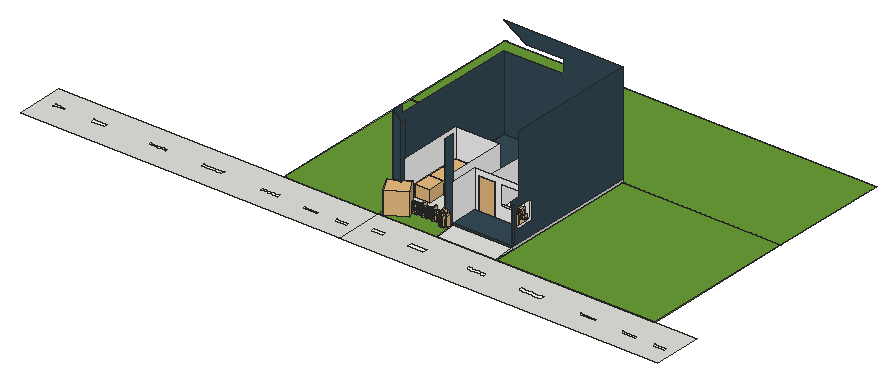
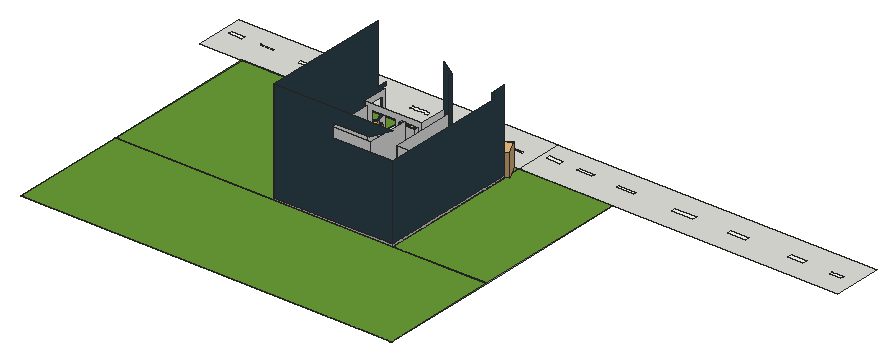
# SketchUp Ruby script. Lengths in inches.
U = 1.inch
M = Sketchup.active_model
def pt(a) = Geom::Point3d.new(a.map { |v| v * U })
def face(e, loops, mat)
  f = e.add_face(loops[0].map { |a| pt(a) })
  loops[1..].each { |l| e.add_face(l.map { |a| pt(a) }).erase! }
  f.material = f.back_material = mat if mat
  f
end
# faces: each face lists its corners as indices into pts; further lists are holes
def faces(e, pts, list, mat = nil) = list.each { |f| face(e, (f[0].is_a?(Array) ? f : [f]).map { |l| l.map { |i| pts[i] } }, mat) }
# xy, xz, yz: faces in a plane at the given z, y or x. An outline is a flat list of corners, or four numbers for a rectangle; further outlines are holes
def ring(l) = l.size == 4 ? [[l[0], l[1]], [l[2], l[1]], [l[2], l[3]], [l[0], l[3]]] : l.each_slice(2).to_a
def flat(e, list, mat, &to3) = list.each { |f| face(e, (f[0].is_a?(Array) ? f : [f]).map { |l| ring(l).map { |u, v| to3.(u, v) } }, mat) }
def xy(e, z, list, mat = nil) = flat(e, list, mat) { |x, y| [x, y, z] }
def xz(e, y, list, mat = nil) = flat(e, list, mat) { |x, z| [x, y, z] }
def yz(e, x, list, mat = nil) = flat(e, list, mat) { |y, z| [x, y, z] }
def lines(e, pts, list) = list.each { |a, b| e.add_line(pt(pts[a]), pt(pts[b])) }
# prism: a flat outline (further loops are holes) pulled along v
def prism(e, loops, v, mat = nil)
  f = face(e, loops, mat); d = Geom::Vector3d.new(v.map { |x| x * U })
  f.pushpull(f.normal.samedirection?(d) ? d.length : -d.length)
end
def box(e, o, s, mat = nil) = prism(e, [[o, [o[0] + s[0], o[1], o[2]], [o[0] + s[0], o[1] + s[1], o[2]], [o[0], o[1] + s[1], o[2]]]], [0, 0, s[2]], mat)
def at(x, y, z, deg = 0) = Geom::Transformation.translation(pt([x, y, z])) * Geom::Transformation.rotation(ORIGIN, Z_AXIS, deg.degrees)
def axes(o, x, y, z) = Geom::Transformation.new([*x, 0, *y, 0, *z, 0, *pt(o).to_a, 1])
def part(name) = M.definitions.add(name)
# library, detail: a bought-in or finely detailed component or shape, given as its bounding box
def library(name, o, s) = part(name).tap { |d| box(d.entities, o, s) }
def detail(e, o, s) = box(e.add_group.entities, o, s)
def put(e, d, t, mat = nil) = e.add_instance(d, t).tap { |i| i.material = mat if mat }
def group(e, t, mat = nil) = e.add_group.tap { |g| g.transformation = t; g.material = mat if mat }.entities
root = M.entities
M.materials.add("0496 AP 9691 Shadow-N").color = [53, 75, 86]
M.materials.add("Color_1").color = [255, 255, 255]
M.materials.add("POT_TEXTURE_1").color = [172, 172, 172]
M.materials.add("[Color M00]").color = [255, 255, 255]
M.materials.add("[Grass Dark Green]").color = [106, 157, 55]
M.materials.add("skp avat flo 1").color = [0, 129, 229]
M.materials.add("skp avat flo 2").color = [47, 120, 22]
M.materials.add("soil1").color = [68, 55, 47]
c1 = library("ruselia",[-5.83,-15.14,-32.53],[55.24,20.14,57.16])
c2 = part("Untitled")
xy(c2.entities,0,[[[158.81,26.5625,306.06,993.3125],[226.57,518.17,239.57,583.92],[225.28,357.51,237.28,411.51],[222.61,182.28,236.36,226.53],[239.71,931.55,251.46,972.3],[233.64,703.93,242.14,755.18],[240.05,835.03,248.8,880.53],[222.04,66.5,231.29,100.5]]])
xy(c2.entities,0,[[222.04,66.5,231.29,100.5],[222.61,182.28,236.36,226.53],[225.28,357.51,237.28,411.51],[226.57,518.17,239.57,583.92],[233.64,703.93,242.14,755.18],
  [240.05,835.03,248.8,880.53],[239.71,931.55,251.46,972.3]],"Color_1")
c3 = library("Cay chuoi",[-26.05,-21.66,0],[63.57,52.43,69.02])
c4 = library("Group\#146",[-640.625,-1318.37,287.11],[396.64,314.81,689.96])
c5 = library("Group\#133",[-513.94,-1201.2,195.17],[480.66,557.42,1160.08])
c6 = library("Group\#135",[-208.03,-1336.63,286.21],[381.72,484.79,1145.39])
c7 = library("Group\#149",[-619.83,-1636.3,288.9],[316.15,456.61,1171.28])
c8 = library("Group\#150",[-738.91,-1210.08,301],[426.4,388.88,1000.79])
c9 = library("Group\#152",[-208.33,-1511.76,297.04],[508.2,421.96,1258.76])
c10 = library("Group\#134",[-545.36,-1775.03,287.125],[412.21,432,920.68])
c11 = library("Group\#147",[-750.24,-1478.51,301.56],[423.84,451.05,998.69])
c12 = library("Group\#137",[-245.33,-1174.2,301.22],[356.02,306.31,608.34])
c13 = library("Group\#132",[-487.23,-1483.58,-4.71],[450.86,446.99,418.38])
c14 = library("Group\#154",[-445.7,-1606.55,154.18],[255.44,283.57,849.28])
c15 = library("Group\#155",[-390.1,-1177.12,195.59],[220.93,265.44,790.12])
c16 = library("Group\#157",[-480.32,-1333.42,295.8],[424.49,356.06,1482.77])
c17 = library("Group\#158",[-378.01,-1245.98,305.66],[422.15,474.55,1267.42])
c18 = library("Group\#136",[-163.65,-1622.09,292.29],[406.18,374.8,780.12])
c19 = library("Group\#153",[-384.8,-1640.99,300.61],[422.68,348.03,1297.96])
c20 = library("Group\#131",[-373.85,-1441.17,362.05],[290.51,348.28,45.35])
c21 = library("Group\#156",[-208.0625,-1498.77,286.27],[547.26,435.76,1075.6])
c22 = library("Group\#151",[-172.82,-1329.68,294.68],[502.85,397.72,955.79])
c23 = library("Group\#148",[-426.76,-1753.59,287.48],[479.67,412.35,1049.19])
c24 = part("Potted palm")
put(c24.entities,c4,axes([750.24,1775.03,-132.93],[1,0,0],[0,1,0],[0,0,1.2036]))
put(c24.entities,c5,axes([750.24,1775.03,-132.93],[1,0,0],[0,1,0],[0,0,1.2036]))
put(c24.entities,c6,axes([750.24,1775.03,-132.93],[1,0,0],[0,1,0],[0,0,1.2036]))
put(c24.entities,c7,axes([750.24,1775.03,-132.93],[1,0,0],[0,1,0],[0,0,1.2036]))
put(c24.entities,c8,axes([750.24,1775.03,-132.93],[1,0,0],[0,1,0],[0,0,1.2036]))
put(c24.entities,c9,axes([750.24,1775.03,-132.93],[1,0,0],[0,1,0],[0,0,1.2036]))
put(c24.entities,c10,axes([750.24,1775.03,-132.93],[1,0,0],[0,1,0],[0,0,1.2036]))
put(c24.entities,c11,axes([750.24,1775.03,-132.93],[1,0,0],[0,1,0],[0,0,1.2036]))
put(c24.entities,c12,axes([750.24,1775.03,-132.93],[1,0,0],[0,1,0],[0,0,1.2036]))
put(c24.entities,c13,axes([746.24,1775.03,3.02],[0.89,0,0],[0,1,0],[0,0,0.64]),"POT_TEXTURE_1")
put(c24.entities,c14,axes([750.24,1775.03,-132.93],[1,0,0],[0,1,0],[0,0,1.2036]))
put(c24.entities,c15,axes([750.24,1775.03,-132.93],[1,0,0],[0,1,0],[0,0,1.2036]))
put(c24.entities,c16,axes([750.24,1775.03,-132.93],[1,0,0],[0,1,0],[0,0,1.2036]))
put(c24.entities,c17,axes([750.24,1775.03,-132.93],[1,0,0],[0,1,0],[0,0,1.2036]))
put(c24.entities,c18,axes([750.24,1775.03,-132.93],[1,0,0],[0,1,0],[0,0,1.2036]))
put(c24.entities,c19,axes([750.24,1775.03,-132.93],[1,0,0],[0,1,0],[0,0,1.2036]))
put(c24.entities,c20,at(750.24,1775.03,-101.54),"soil1")
put(c24.entities,c21,axes([750.24,1775.03,-132.93],[1,0,0],[0,1,0],[0,0,1.2036]))
put(c24.entities,c22,axes([750.24,1775.03,-132.93],[1,0,0],[0,1,0],[0,0,1.2036]))
put(c24.entities,c23,axes([750.24,1775.03,-132.93],[1,0,0],[0,1,0],[0,0,1.2036]))
c25 = library("skpD0I6a8",[14.43,-68.68,0],[105.42,143.14,64.75])
c26 = library("skp0QfVtK",[14.45,-36.06,-0.05],[111.77,111,64.8])
c27 = library("skpcyxm1p",[14.43,-75.28,0],[105.19,111.11,34.48])
c28 = library("Sectional sofa module",[0,0,0],[105.41,111.76,64.75])
c29 = part("L Shaped Sofa (30)")
put(c29.entities,c25,at(757.73,0.41,0))
put(c29.entities,c26,axes([685.96,0.19,0],[-1,0,0],[0,1,0],[0,0,1]))
put(c29.entities,c27,at(605.64,-125.1875,0))
put(c29.entities,c28,axes([669.02,-36.11,0],[1,0,0],[0,0.99,0],[0,0,1]))
c30 = library("Group\#97",[-662.41,217.3,320.04],[397.32,658.3,1732.06])
c31 = library("Group\#99",[-299.2,181.55,262.58],[360.65,735.71,1258.34])
c32 = library("Group\#94",[-1038.76,656.55,345.34],[733.18,460.51,2065.7])
c33 = library("Group\#92",[-445.29,890.31,329.28],[284.3,304.08,2023.29])
c34 = library("Group\#95",[-733.48,439.625,202.64],[456.28,533.12,1536.78])
c35 = library("Group\#98",[-455.56,899.32,410.78],[341.21,610.33,1581.5])
c36 = library("Group\#91",[-516.34,626.77,-4.5625],[517.73,515.95,418.98])
c37 = library("Group\#96",[-249.24,914.85,310.18],[345.55,647.95,1307.93])
c38 = library("Group\#93",[-277.97,488.68,287.26],[362.84,405.94,1768.54])
c39 = library("Group\#90",[-468.76,669.89,380.1875],[424.36,427.47,41.99])
c40 = part("Potted tropical plant")
put(c40.entities,c30,at(1038.76,-181.55,4.5625))
put(c40.entities,c31,at(1038.76,-181.55,4.5625))
put(c40.entities,c32,at(1038.76,-181.55,4.5625))
put(c40.entities,c33,at(1038.76,-181.55,4.5625))
put(c40.entities,c34,at(1038.76,-181.55,4.5625))
put(c40.entities,c35,at(1038.76,-181.55,4.5625))
put(c40.entities,c36,at(1038.76,-181.55,4.5625),"POT_TEXTURE_1")
put(c40.entities,c37,at(1038.76,-181.55,4.5625))
put(c40.entities,c38,at(1038.76,-181.55,4.5625))
put(c40.entities,c39,at(1038.76,-181.55,4.5625),"soil1")
c41 = library("door by lz",[5.91,-4.92,0],[35.43,6.61,78.74])
c42 = part("Gruppe\#2")
xy(c42.entities,0,[[6.69,0,4.96,0.23,3.03,1.59,1.96,1.96,0.9,3.35,0.9,5.71,0,6.69,0.23,8.43,1.96,10,3.35,12.49,4.67,13.04,7.04,12.49,8.72,13.04,10.04,12.49,11.43,11.43,12.05,9.15,13.39,6.69,13.16,4.96,12.49,3.35,10.41,2.22,8.43,0.23]],"skp avat flo 1")
c43 = part("Gruppe\#12")
xy(c43.entities,0,[[1.18,0.5,1.36,0.52,1.52,0.59,1.67,0.7,1.77,0.84,1.84,1,1.87,1.18,1.84,1.36,1.77,1.52,1.67,1.67,1.52,1.77,1.36,1.84,1.18,1.87,1,1.84,0.84,1.77,0.7,1.67,0.59,1.52,0.52,1.36,0.5,1.18,0.52,1,0.59,0.84,0.7,0.7,0.84,0.59,1,0.52]])
c44 = part("f.st. wop plant 01 blüte")
put(c44.entities,c42,at(0,0,0))
put(c44.entities,c43,at(5.65,5.41,0.39))
c45 = part("Gruppe\#5")
xy(c45.entities,0.96,[[13.97,0.22,8.73,4.42,7.37,10.11,8.43,14.53,13.97,16.39]],"skp avat flo 2")
p = [[13.97,0.22,0.96],[13.97,16.39,0.96],[17.89,14.53,4.875],[18.64,10.11,5.625],[17.67,4.42,4.66]]
faces(c45.entities,p,[[0,1,2,3,4]],"skp avat flo 2")
c46 = part("f.st. wop plant 01 blatt")
put(c46.entities,c45,axes([0.99,0,4.74],[0.91566,0,-0.40195],[0,1,0],[0.40195,0,0.91566]))
c47 = part("Gruppe\#10")
put(c47.entities,c44,axes([4.61,0.45,57.14],[0.99373,-0.06775,-0.08889],[0.11172,0.62588,0.77188],[0.00335,-0.77697,0.62953]))
put(c47.entities,c44,axes([12.4,0.4,0.59],[0.70061,0.70799,-0.08889],[-0.40079,0.49353,0.77188],[0.59035,-0.50516,0.62953]))
put(c47.entities,c44,axes([24.4375,6.09,17.58],[-0.05734,0.99439,-0.08889],[-0.63495,0.03239,0.77188],[0.77043,0.1007,0.62953]))
put(c47.entities,c44,axes([1.11,8.09,13.25],[0.88983,-0.44754,-0.08889],[0.34553,0.53368,0.77188],[-0.298,-0.71756,0.62953]))
put(c47.entities,c44,axes([23.26,15,37.53],[-0.84836,0.52191,-0.08889],[-0.38985,-0.50222,0.77188],[0.35821,0.68948,0.62953]))
put(c47.entities,c44,axes([12.67,23.61,24.88],[-0.75852,-0.64555,-0.08889],[0.35717,-0.52596,0.77188],[-0.54504,0.55374,0.62953]))
put(c47.entities,c44,axes([20.43,22.9,81.42],[-0.98432,0.15238,-0.08889],[-0.16477,-0.61405,0.77188],[0.06303,0.77442,0.62953]))
put(c47.entities,c44,axes([1.76,2.9,29.21],[0.93833,-0.33412,-0.08889],[0.27691,0.5723,0.77188],[-0.20703,-0.74889,0.62953]))
put(c47.entities,c44,axes([13.59,0.5,77.09],[0.62412,0.77625,-0.08889],[-0.4494,0.44972,0.77188],[0.63915,-0.4418,0.62953]))
put(c47.entities,c44,axes([-1.26,15.51,69.79],[0.24265,-0.96603,-0.08889],[0.62977,0.08716,0.77188],[-0.73791,-0.24328,0.62953]))
put(c47.entities,c44,axes([22.04,17.92,65.46],[-0.95793,0.27287,-0.08889],[-0.2394,-0.58898,0.77188],[0.15827,0.76069,0.62953]))
put(c47.entities,c44,axes([9.51,23.35,52.81],[-0.55554,-0.82673,-0.08889],[0.48617,-0.40969,0.77188],[-0.67455,0.38559,0.62953]))
put(c47.entities,c44,axes([0.1875,18.97,41.86],[-0.02781,-0.99565,-0.08889],[0.62986,-0.08651,0.77188],[-0.77621,-0.03452,0.62953]))
put(c47.entities,c44,axes([24.98,7.4,94.08],[-0.15925,0.98323,-0.08889],[-0.63491,-0.03305,0.77188],[0.75599,0.17936,0.62953]))
put(c47.entities,c44,axes([21.5,21.98,4.93],[-0.96344,0.25275,-0.08889],[-0.22702,-0.59386,0.77188],[0.1423,0.76384,0.62953]))
put(c47.entities,c44,axes([1.57,6.98,89.75],[0.93112,-0.3537,-0.08889],[0.28884,0.56637,0.77188],[-0.22267,-0.74439,0.62953]))
put(c47.entities,c46,axes([9.37,32.32,90.95],[-0.51317,-0.65235,0],[0.5996,-0.47167,0.32697],[-0.25699,0.20216,0.76288]))
put(c47.entities,c46,axes([33.81,6.72,78.35],[-0.27992,0.78137,0],[-0.71819,-0.25729,0.32697],[0.30782,0.11027,0.76288]))
put(c47.entities,c46,axes([-9.46,14.86,61.47],[0.53029,-0.63851,0],[0.58688,0.4874,0.32697],[-0.25154,-0.2089,0.76288]))
put(c47.entities,c46,axes([21.49,-6.15,66.98],[0.2591,0.78852,0],[-0.72476,0.23815,0.32697],[0.31063,-0.10207,0.76288]))
put(c47.entities,c46,axes([32.03,5.27,54.38],[-0.36397,0.74594,0],[-0.68562,-0.33454,0.32697],[0.29386,0.14338,0.76288]))
put(c47.entities,c46,axes([30.63,20.6,49.31],[-0.77544,0.29596,0],[-0.27203,-0.71273,0.32697],[0.11659,0.30548,0.76288]))
put(c47.entities,c46,axes([32.03,5.27,27.16],[-0.36397,0.74594,0],[-0.68562,-0.33454,0.32697],[0.29386,0.14338,0.76288]))
put(c47.entities,c46,axes([17.4375,27.53,13.8125],[-0.76735,-0.23527,0.21148],[0.29408,-0.735,0.24937],[0.11659,0.30548,0.76288]))
put(c47.entities,c46,axes([-9.46,14.86,34.24],[0.53029,-0.63851,0],[0.58688,0.4874,0.32697],[-0.25154,-0.2089,0.76288]))
c48 = part("Gruppe\#9")
put(c48.entities,c44,axes([2.2,1.62,57.61],[0.97169,-0.0623,-0.22792],[0.22172,0.57378,0.78843],[0.08166,-0.81664,0.57134]))
put(c48.entities,c44,axes([-1.48,7.53,1.27],[0.68093,0.71536,-0.15682],[-0.22028,0.40428,0.88771],[0.69843,-0.56993,0.43287]))
put(c48.entities,c44,axes([13.97,11.34,15.86],[-0.0542,0.99797,0.03349],[-0.45869,-0.05467,0.88691],[0.88694,0.03271,0.46072]))
put(c48.entities,c44,axes([-9.71,13.74,16.77],[0.84218,-0.4326,-0.32186],[0.5102,0.4462,0.73526],[-0.17446,-0.78343,0.59649]))
put(c48.entities,c44,axes([17.17,17.99,36.46],[-0.83727,0.52624,0.14846],[-0.23006,-0.58536,0.77745],[0.49603,0.61679,0.61117]))
put(c48.entities,c44,axes([4.35,27.92,27.32],[-0.77345,-0.63385,0.00301],[0.4998,-0.60694,0.61792],[-0.38984,0.47943,0.78623]))
put(c48.entities,c44,axes([20.43,22.9,81.42],[-0.98432,0.15238,-0.08889],[-0.16477,-0.61405,0.77188],[0.06303,0.77442,0.62953]))
put(c48.entities,c44,axes([-5.84,6.82,31.58],[0.89192,-0.31974,-0.31975],[0.44391,0.4844,0.75386],[-0.08616,-0.81432,0.57398]))
put(c48.entities,c44,axes([13.59,0.5,77.09],[0.62412,0.77625,-0.08889],[-0.4494,0.44972,0.77188],[0.63915,-0.4418,0.62953]))
put(c48.entities,c44,axes([-1.26,15.51,69.79],[0.24265,-0.96603,-0.08889],[0.62977,0.08716,0.77188],[-0.73791,-0.24328,0.62953]))
put(c48.entities,c44,axes([20.77,18.5,64.59],[-0.95848,0.27864,0.06062],[-0.13765,-0.63827,0.75741],[0.24973,0.71762,0.65012]))
put(c48.entities,c44,axes([6.6875,24.75,54.15],[-0.57029,-0.8188,-0.06577],[0.58283,-0.45976,0.67002],[-0.57885,0.34377,0.73942]))
put(c48.entities,c44,axes([-4.08,21.11,44.3125],[-0.04911,-0.98765,-0.14878],[0.72825,-0.13735,0.67141],[-0.68355,-0.07538,0.726]))
put(c48.entities,c44,axes([24.98,7.4,94.08],[-0.15925,0.98323,-0.08889],[-0.63491,-0.03305,0.77188],[0.75599,0.17936,0.62953]))
put(c48.entities,c44,axes([8.77,28.52,5.9],[-0.95532,0.25842,0.14346],[-0.07274,-0.676,0.7333],[0.28648,0.6901,0.6646]))
put(c48.entities,c44,axes([1.57,6.98,89.75],[0.93112,-0.3537,-0.08889],[0.28884,0.56637,0.77188],[-0.22267,-0.74439,0.62953]))
put(c48.entities,c46,axes([9.37,32.32,90.95],[-0.51317,-0.65235,0],[0.5996,-0.47167,0.32697],[-0.25699,0.20216,0.76288]))
put(c48.entities,c46,axes([33.81,6.72,78.35],[-0.27992,0.78137,0],[-0.71819,-0.25729,0.32697],[0.30782,0.11027,0.76288]))
put(c48.entities,c46,axes([-11.01,15.72,64.74],[0.51926,-0.63742,-0.11388],[0.63054,0.46456,0.27478],[-0.14729,-0.25842,0.77487]))
put(c48.entities,c46,axes([20.21,-5.625,64.6],[0.26417,0.78668,0.01588],[-0.67119,0.21655,0.43762],[0.41063,-0.15212,0.70508]))
put(c48.entities,c46,axes([29.04,6.59,51.45],[-0.35348,0.74452,0.09816],[-0.63785,-0.35493,0.39506],[0.39635,0.09281,0.72332]))
put(c48.entities,c46,axes([27.11,22.23,47.625],[-0.76537,0.29574,0.12508],[-0.23173,-0.73252,0.31403],[0.22228,0.25465,0.75805]))
put(c48.entities,c46,axes([23.375,9.49,23.48],[-0.34051,0.7404,0.15735],[-0.60881,-0.37042,0.42548],[0.44978,0.05914,0.69506]))
put(c48.entities,c46,axes([6.77,33.04,15.99],[-0.71083,-0.25923,0.3412],[0.32455,-0.75723,0.10082],[0.2798,0.21977,0.74988]))
put(c48.entities,c46,axes([-15.51,18.125,40.12],[0.50532,-0.63318,-0.18065],[0.65217,0.44994,0.24724],[-0.09068,-0.29247,0.77145]))
c49 = part("Gruppe\#11")
put(c49.entities,c44,axes([4.61,0.45,57.14],[0.99373,-0.06775,-0.08889],[0.11172,0.62588,0.77188],[0.00335,-0.77697,0.62953]))
put(c49.entities,c44,axes([12.4,0.4,0.59],[0.70061,0.70799,-0.08889],[-0.40079,0.49353,0.77188],[0.59035,-0.50516,0.62953]))
put(c49.entities,c44,axes([24.4375,6.09,17.58],[-0.05734,0.99439,-0.08889],[-0.63495,0.03239,0.77188],[0.77043,0.1007,0.62953]))
put(c49.entities,c44,axes([1.11,8.09,13.25],[0.88983,-0.44754,-0.08889],[0.34553,0.53368,0.77188],[-0.298,-0.71756,0.62953]))
put(c49.entities,c44,axes([23.26,15,37.53],[-0.84836,0.52191,-0.08889],[-0.38985,-0.50222,0.77188],[0.35821,0.68948,0.62953]))
put(c49.entities,c44,axes([12.67,23.61,24.88],[-0.75852,-0.64555,-0.08889],[0.35717,-0.52596,0.77188],[-0.54504,0.55374,0.62953]))
put(c49.entities,c44,axes([20.43,22.9,81.42],[-0.98432,0.15238,-0.08889],[-0.16477,-0.61405,0.77188],[0.06303,0.77442,0.62953]))
put(c49.entities,c44,axes([1.76,2.9,29.21],[0.93833,-0.33412,-0.08889],[0.27691,0.5723,0.77188],[-0.20703,-0.74889,0.62953]))
put(c49.entities,c44,axes([13.59,0.5,77.09],[0.62412,0.77625,-0.08889],[-0.4494,0.44972,0.77188],[0.63915,-0.4418,0.62953]))
put(c49.entities,c44,axes([-1.26,15.51,69.79],[0.24265,-0.96603,-0.08889],[0.62977,0.08716,0.77188],[-0.73791,-0.24328,0.62953]))
put(c49.entities,c44,axes([22.04,17.92,65.46],[-0.95793,0.27287,-0.08889],[-0.2394,-0.58898,0.77188],[0.15827,0.76069,0.62953]))
put(c49.entities,c44,axes([9.51,23.35,52.81],[-0.55554,-0.82673,-0.08889],[0.48617,-0.40969,0.77188],[-0.67455,0.38559,0.62953]))
put(c49.entities,c44,axes([0.1875,18.97,41.86],[-0.02781,-0.99565,-0.08889],[0.62986,-0.08651,0.77188],[-0.77621,-0.03452,0.62953]))
put(c49.entities,c44,axes([24.98,7.4,94.08],[-0.15925,0.98323,-0.08889],[-0.63491,-0.03305,0.77188],[0.75599,0.17936,0.62953]))
put(c49.entities,c44,axes([21.5,21.98,4.93],[-0.96344,0.25275,-0.08889],[-0.22702,-0.59386,0.77188],[0.1423,0.76384,0.62953]))
put(c49.entities,c44,axes([1.57,6.98,89.75],[0.93112,-0.3537,-0.08889],[0.28884,0.56637,0.77188],[-0.22267,-0.74439,0.62953]))
put(c49.entities,c46,axes([9.37,32.32,90.95],[-0.51317,-0.65235,0],[0.5996,-0.47167,0.32697],[-0.25699,0.20216,0.76288]))
put(c49.entities,c46,axes([33.81,6.72,78.35],[-0.27992,0.78137,0],[-0.71819,-0.25729,0.32697],[0.30782,0.11027,0.76288]))
put(c49.entities,c46,axes([-9.46,14.86,61.47],[0.53029,-0.63851,0],[0.58688,0.4874,0.32697],[-0.25154,-0.2089,0.76288]))
put(c49.entities,c46,axes([21.49,-6.15,66.98],[0.2591,0.78852,0],[-0.72476,0.23815,0.32697],[0.31063,-0.10207,0.76288]))
put(c49.entities,c46,axes([32.03,5.27,54.38],[-0.36397,0.74594,0],[-0.68562,-0.33454,0.32697],[0.29386,0.14338,0.76288]))
put(c49.entities,c46,axes([30.63,20.6,49.31],[-0.77544,0.29596,0],[-0.27203,-0.71273,0.32697],[0.11659,0.30548,0.76288]))
put(c49.entities,c46,axes([32.03,5.27,27.16],[-0.36397,0.74594,0],[-0.68562,-0.33454,0.32697],[0.29386,0.14338,0.76288]))
put(c49.entities,c46,axes([17.4375,27.53,13.8125],[-0.76735,-0.23527,0.21148],[0.29408,-0.735,0.24937],[0.11659,0.30548,0.76288]))
put(c49.entities,c46,axes([-9.46,14.86,34.24],[0.53029,-0.63851,0],[0.58688,0.4874,0.32697],[-0.25154,-0.2089,0.76288]))
c50 = part("Gruppe\#8")
put(c50.entities,c44,axes([2.26,1.13,59.39],[0.92531,-0.05375,-0.37538],[0.3384,0.56379,0.75341],[0.17114,-0.82417,0.53987]))
put(c50.entities,c44,axes([-9.39,6.25,4.33],[0.64151,0.72107,-0.26176],[-0.09814,0.41557,0.90425],[0.76081,-0.5544,0.33735]))
put(c50.entities,c44,axes([7.9,10.48,16.53],[-0.06325,0.99763,0.02691],[-0.32763,-0.04623,0.94367],[0.94269,0.05087,0.32978]))
put(c50.entities,c44,axes([-15.4375,12.6,20.76],[0.79424,-0.42729,-0.43198],[0.60271,0.46401,0.64918],[-0.07695,-0.77596,0.62607]))
put(c50.entities,c44,axes([13.9,17.49,36.37],[-0.81529,0.51823,0.25834],[-0.1092,-0.57574,0.81031],[0.56867,0.63242,0.52599]))
put(c50.entities,c44,axes([-0.23,27.12,29.01],[-0.75604,-0.64315,0.1215],[0.59094,-0.59091,0.5492],[-0.28142,0.48702,0.82681]))
put(c50.entities,c44,axes([20.43,22.9,81.42],[-0.98432,0.15238,-0.08889],[-0.16477,-0.61405,0.77188],[0.06303,0.77442,0.62953]))
put(c50.entities,c44,axes([-9.41,5.97,34.96],[0.84215,-0.31382,-0.43852],[0.53918,0.50168,0.67646],[0.00771,-0.80612,0.5917]))
put(c50.entities,c44,axes([13.59,0.5,77.09],[0.62412,0.77625,-0.08889],[-0.4494,0.44972,0.77188],[0.63915,-0.4418,0.62953]))
put(c50.entities,c44,axes([-1.26,15.51,69.79],[0.24265,-0.96603,-0.08889],[0.62977,0.08716,0.77188],[-0.73791,-0.24328,0.62953]))
put(c50.entities,c44,axes([22.04,17.92,65.46],[-0.95793,0.27287,-0.08889],[-0.2394,-0.58898,0.77188],[0.15827,0.76069,0.62953]))
put(c50.entities,c44,axes([6.08,24.33,55.62],[-0.57097,-0.82091,0.01051],[0.68037,-0.46598,0.56565],[-0.45945,0.33012,0.82458]))
put(c50.entities,c44,axes([-6.06,20.77,47.51],[-0.06819,-0.9857,-0.15407],[0.82323,-0.14283,0.54945],[-0.56361,-0.08937,0.8212]))
put(c50.entities,c44,axes([24.98,7.4,94.08],[-0.15925,0.98323,-0.08889],[-0.63491,-0.03305,0.77188],[0.75599,0.17936,0.62953]))
put(c50.entities,c44,axes([1.11,27.4375,7.17],[-0.92899,0.24893,0.27387],[0.04156,-0.66514,0.74556],[0.36776,0.70401,0.60756]))
put(c50.entities,c44,axes([1.57,6.98,89.75],[0.93112,-0.3537,-0.08889],[0.28884,0.56637,0.77188],[-0.22267,-0.74439,0.62953]))
put(c50.entities,c46,axes([9.37,32.32,90.95],[-0.51317,-0.65235,0],[0.5996,-0.47167,0.32697],[-0.25699,0.20216,0.76288]))
put(c50.entities,c46,axes([33.81,6.72,78.35],[-0.27992,0.78137,0],[-0.71819,-0.25729,0.32697],[0.30782,0.11027,0.76288]))
put(c50.entities,c46,axes([-9.74,15.05,68.68],[0.49765,-0.63289,-0.20172],[0.66377,0.46408,0.1815],[-0.02561,-0.27014,0.78439]))
put(c50.entities,c46,axes([21.49,-6.15,66.98],[0.2591,0.78852,0],[-0.72476,0.23815,0.32697],[0.31063,-0.10207,0.76288]))
put(c50.entities,c46,axes([27.8125,6.34,49.26],[-0.33661,0.74111,0.1623],[-0.5684,-0.36396,0.48306],[0.5025,0.08476,0.65514]))
put(c50.entities,c46,axes([25.26,22.01,46],[-0.73801,0.28975,0.24554],[-0.17833,-0.73814,0.33502],[0.33532,0.24514,0.71859]))
put(c50.entities,c46,axes([18.32,8.86,22.77],[-0.32541,0.73857,0.19371],[-0.53703,-0.37106,0.51265],[0.54278,0.07565,0.62335]))
put(c50.entities,c46,axes([0.49,32.09,17.38],[-0.65154,-0.26248,0.44214],[0.34641,-0.75151,0.06433],[0.37999,0.23503,0.69948]))
put(c50.entities,c46,axes([-17.94,17.29,44.63],[0.48369,-0.62973,-0.24163],[0.67408,0.46176,0.14595],[0.0237,-0.2813,0.78052]))
c51 = part("f.st. wop plant 01")
put(c51.entities,c47,at(39.14,64.09,18.66,-141.2))
put(c51.entities,c48,axes([53.54,120.93,12.24],[-0.61849,0.75929,0.20233],[-0.78178,-0.62056,-0.06099],[0.07925,-0.1959,0.97742]))
put(c51.entities,c49,at(82.26,36.89,18.66))
put(c51.entities,c50,axes([72.55,-5.87,29.3],[0.62579,-0.70508,0.33355],[0.76326,0.64164,-0.07566],[-0.16067,0.30193,0.93969]))
c52 = part("World of Pandora - tree 01")
put(c52.entities,c51,at(57.06,8.63,0))
xy(root,0,[[679.74,147.25,964.11,627.5625],[964.11,627.3125,964.11,627.5625,679.72,627.5625,679.72,987.25,1804.17,987.25,1804.17,627.3125]],"[Grass Dark Green]")
xy(root,1,[[679.74,147.25,964.11,147.25,964.11,627.3125,681.55,627.3125,679.74,627.51,679.72,627.5625,679.74,627.5625],[964.11,627.3125,1804.17,627.3125,1804.17,987.25,679.72,987.25,679.72,627.5625,964.11,627.5625],[681.55,627.3125,964.11,627.3125,964.11,627.5625,679.74,627.5625,679.74,627.51],[679.74,627.51,679.74,627.5625,679.72,627.5625]],"[Grass Dark Green]")
xy(root,7,[[964.11,207.25,964.11,627.25,1324.11,627.25,1324.11,207.25,1120.11,207.25,1120.11,414.75,988.11,414.75,988.11,220.25,965.96,207.25],[965.96,207.25,988.11,220.25,988.11,207.25]],"0496 AP 9691 Shadow-N")
xy(root,13,[[1144.11,207.25,1324.11,207.25,1324.11,217.8125,1316.11,217.8125,1316.11,291.25,1204.42,291.25,1204.42,299.25,1187.61,299.25,1187.61,303.3125,1156.42,303.3125,1156.42,291.25,1144.11,291.25],[1187.61,299.25,1204.42,303.3125]],"0496 AP 9691 Shadow-N")
xy(root,13,[[1204.42,299.25,1304.61,299.25,1304.61,429.625,1187.61,429.625,1187.61,303.3125,1204.42,303.3125]],"[Color M00]")
xz(root,147.25,[[679.74,0,964.11,1]])
xz(root,207.25,[[964.11,7,988.11,7,988.11,231,964.11,255],[1120.11,7,1144.11,7,1144.11,255,1120.11,231],[1144.11,7,1324.11,13]],"0496 AP 9691 Shadow-N")
xz(root,217.8125,[[1316.11,13,1324.11,125]],"0496 AP 9691 Shadow-N")
xz(root,291.25,[[[1144.11,13,1156.42,13,1156.42,109,1204.42,109,1204.42,13,1316.11,13,1316.11,125,1144.11,125],[1223.61,49,1295.36,109]]],"[Color M00]")
xz(root,299.25,[[1187.61,13,1304.61,49]],"[Color M00]")
xz(root,303.3125,[[1156.42,13,1204.42,109]],"[Color M00]")
xz(root,414.75,[[988.11,7,1120.11,127]],"[Color M00]")
xz(root,429.625,[[1187.61,13,1304.61,118.25]],"[Color M00]")
xz(root,627.25,[[964.11,7,964.11,232.625,1144.11,232.625,1144.11,272.98,1032.78,272.98,964.11,315,1324.11,315,1324.11,7]],"0496 AP 9691 Shadow-N")
xz(root,627.3125,[[964.11,0,1804.17,1]],"[Grass Dark Green]")
xz(root,627.5625,[[679.74,0,964.11,1]])
xz(root,627.5625,[[679.72,0,679.74,1]],"[Grass Dark Green]")
xz(root,987.25,[[679.72,0,1804.17,1]],"[Grass Dark Green]")
yz(root,679.72,[[627.5625,0,987.25,1]],"[Grass Dark Green]")
yz(root,679.74,[[147.25,0,627.5625,1]])
yz(root,964.11,[[147.25,0,627.3125,1]])
yz(root,964.11,[[207.25,7,207.25,255,240.97,255,240.97,232.625,627.25,232.625,627.25,7]],"0496 AP 9691 Shadow-N")
yz(root,964.11,[[627.3125,0,627.5625,1]],"[Grass Dark Green]")
yz(root,988.11,[[207.25,7,220.25,7,220.25,127,217.0625,127,217.0625,133,220.25,133,220.25,231,207.25,231]],"0496 AP 9691 Shadow-N")
yz(root,988.11,[[220.25,7,414.75,127]],"[Color M00]")
yz(root,1120.11,[[207.25,7,207.25,231,220.25,231,220.25,133,217.0625,133,217.0625,127,220.25,127,220.25,7]],"0496 AP 9691 Shadow-N")
yz(root,1120.11,[[220.25,7,414.75,127]],"[Color M00]")
yz(root,1144.11,[[207.25,13,291.25,125]],"[Color M00]")
yz(root,1156.42,[[291.25,13,303.3125,109]],"[Color M00]")
yz(root,1187.61,[[299.25,13,429.625,13,429.625,118.25,303.3125,118.25,303.3125,109,299.25,109]],"[Color M00]")
yz(root,1204.42,[[291.25,13,303.3125,109]],"[Color M00]")
yz(root,1304.61,[[299.25,13,429.625,118.25]],"[Color M00]")
yz(root,1316.11,[[[217.8125,13,291.25,125],[234.26,49,272.24,49,275.61,49.31,278.36,50.22,280.5,51.75,282.03,53.89,282.94,56.64,283.25,60.01,283.25,97.99,282.94,101.36,282.03,104.11,280.5,106.25,278.36,107.78,275.61,108.69,272.24,109,234.26,109,230.89,108.69,228.14,107.78,226,106.25,224.47,104.11,223.56,101.36,223.25,97.99,223.25,60.01,223.56,56.64,224.47,53.89,226,51.75,228.14,50.22,230.89,49.31]]],"[Color M00]")
yz(root,1324.11,[[[207.25,7,627.25,7,627.25,315,234.25,315,234.25,135,203.25,135,203.25,125,217.8125,125,217.8125,13,207.25,13],[234.26,49,230.89,49.31,228.14,50.22,226,51.75,224.47,53.89,223.56,56.64,223.25,60.01,223.25,97.99,223.56,101.36,224.47,104.11,226,106.25,228.14,107.78,230.89,108.69,234.26,109,272.24,109,275.61,108.69,278.36,107.78,280.5,106.25,282.03,104.11,282.94,101.36,283.25,97.99,283.25,60.01,282.94,56.64,282.03,53.89,280.5,51.75,278.36,50.22,275.61,49.31,272.24,49]]],"0496 AP 9691 Shadow-N")
yz(root,1804.17,[[627.3125,0,987.25,1]],"[Grass Dark Green]")
p = [[988.11,220.25,7],[965.96,207.25,7]]
lines(root,p,[[0,1]])
g1 = group(root,at(964.11,147.25,0))
xy(g1,0,[[0,0,360,480]])
xy(g1,0,[[360,0,840.0625,480.0625]],"[Grass Dark Green]")
xy(g1,1,[[0,0,180,60],[360,0,840.0625,480.0625]],"[Grass Dark Green]")
xy(g1,7,[[0,60,24,60,24,75,156,75,156,60,360,60,360,480,0,480]])
xy(g1,21.5,[[24,60,156,75]])
xz(g1,0,[[0,0,180,1],[180,0,360,1]])
xz(g1,0,[[360,0,840.0625,1]],"[Grass Dark Green]")
xz(g1,60,[[24,1,156,21.5]])
xz(g1,60,[[0,1,24,7],[156,1,180,7]],"0496 AP 9691 Shadow-N")
xz(g1,75,[[24,7,156,21.5]])
xz(g1,480,[[0,0,360,7]])
xz(g1,480.0625,[[360,0,840.0625,1]],"[Grass Dark Green]")
yz(g1,0,[[0,0,60,1],[60,0,480,7]])
yz(g1,24,[[60,7,75,21.5]])
yz(g1,156,[[60,7,75,21.5]])
yz(g1,180,[[0,1,60,7,60,1]])
yz(g1,360,[[0,1,60,1,60,7],[60,1,480,7]])
yz(g1,360,[[0,0,60,1],[60,0,480,1],[480,0,480.0625,1]],"[Grass Dark Green]")
yz(g1,840.0625,[[0,0,480.0625,1]],"[Grass Dark Green]")
p = [[180,60,7],[180,0,1],[360,0,1],[360,60,7]]
faces(g1,p,[[0,1,2,3]])
put(root,c1,axes([1025.64,206.48,9.02],[0.26962,0.00972,0],[-0.00972,0.26962,0],[0,0,0.2698]))
put(root,c1,axes([1057.07,206.48,9.02],[0.26962,0.00972,0],[-0.00972,0.26962,0],[0,0,0.2698]))
put(root,c1,axes([1085.76,206.48,9.02],[0.26962,0.00972,0],[-0.00972,0.26962,0],[0,0,0.2698]))
put(root,c1,axes([1039.28,206.59,9.13],[0.26962,0.00972,0],[-0.00321,0.08898,0],[0,0,0.2698]))
put(root,c1,axes([1070.72,206.59,9.13],[0.26962,0.00972,0],[-0.00321,0.08898,0],[0,0,0.2698]))
put(root,c1,axes([1099.41,206.59,9.13],[0.26962,0.00972,0],[-0.00321,0.08898,0],[0,0,0.2698]))
put(root,c2,at(937.55,306.06,1,-90))
put(root,c2,at(-26.5625,306.06,1,-90))
put(root,c3,at(991.2,181.98,1,30))
put(root,c24,axes([1114.28,185.97,1],[0.02235,0,0],[0,0.02235,0],[0,0,0.02235]))
put(root,c1,axes([1021.57,204.61,11.23],[0.26962,0.00972,0],[-0.00321,0.08898,0],[0,0,0.2698]))
put(root,c1,axes([1053,204.61,11.23],[0.26962,0.00972,0],[-0.00321,0.08898,0],[0,0,0.2698]))
put(root,c1,axes([1081.69,204.61,11.23],[0.26962,0.00972,0],[-0.00321,0.08898,0],[0,0,0.2698]))
put(root,c1,axes([1033.41,205.89,11.82],[0.26962,0.00972,0],[-0.00321,0.08898,0],[0,0,0.2698]))
put(root,c1,axes([1064.84,205.89,11.82],[0.26962,0.00972,0],[-0.00321,0.08898,0],[0,0,0.2698]))
put(root,c1,axes([1093.53,205.89,11.82],[0.26962,0.00972,0],[-0.00321,0.08898,0],[0,0,0.2698]))
put(root,c1,axes([1009.37,203.92,13.24],[0.26962,0.00972,0],[-0.00321,0.08898,0],[0,0,0.2698]))
put(root,c1,axes([1040.81,203.92,13.24],[0.26962,0.00972,0],[-0.00321,0.08898,0],[0,0,0.2698]))
put(root,c1,axes([1069.5,203.92,13.24],[0.26962,0.00972,0],[-0.00321,0.08898,0],[0,0,0.2698]))
put(root,c1,axes([1025.8,203.24,14.45],[0.26962,0.00972,0],[-0.00321,0.08898,0],[0,0,0.2698]))
put(root,c1,axes([1057.23,203.24,14.45],[0.26962,0.00972,0],[-0.00321,0.08898,0],[0,0,0.2698]))
put(root,c1,axes([1085.92,203.24,14.45],[0.26962,0.00972,0],[-0.00321,0.08898,0],[0,0,0.2698]))
put(root,c29,axes([1021.31,-14.64,6.98],[0,0.4845,0],[-0.4161,0,0],[0,0,0.57]))
put(root,c1,axes([1033.17,206.76,17.01],[0.26962,0.00972,0],[-0.00972,0.26962,0],[0,0,0.2698]))
put(root,c1,axes([1064.61,206.76,17.01],[0.26962,0.00972,0],[-0.00972,0.26962,0],[0,0,0.2698]))
put(root,c1,axes([1093.29,206.76,17.01],[0.26962,0.00972,0],[-0.00972,0.26962,0],[0,0,0.2698]))
put(root,c1,axes([1013.87,203.14,17.93],[0.26962,0.00972,0],[-0.00321,0.08898,0],[0,0,0.2698]))
put(root,c1,axes([1045.3,203.14,17.93],[0.26962,0.00972,0],[-0.00321,0.08898,0],[0,0,0.2698]))
put(root,c1,axes([1073.99,203.14,17.93],[0.26962,0.00972,0],[-0.00321,0.08898,0],[0,0,0.2698]))
put(root,c1,axes([1044.23,205.97,19.78],[0.15908,0.00574,0],[-0.00321,0.08898,0],[0,0,0.2698]))
put(root,c1,axes([1075.67,205.97,19.78],[0.15908,0.00574,0],[-0.00321,0.08898,0],[0,0,0.2698]))
put(root,c1,axes([1104.35,205.97,19.78],[0.15908,0.00574,0],[-0.00321,0.08898,0],[0,0,0.2698]))
put(root,c40,axes([1273.25,288.08,13],[0.00626,-0.02338,0],[0.02338,0.00626,0],[0,0,0.0242]))
put(root,c41,axes([1148.42,296.17,13],[1.35467,0,0],[0,1,0],[0,0,1.2192]),"0496 AP 9691 Shadow-N")
put(root,c1,axes([997.82,205.29,22.09],[0.26962,0.00972,0],[-0.00972,0.26962,0],[0,0,0.2698]))
put(root,c1,axes([1029.26,205.29,22.09],[0.26962,0.00972,0],[-0.00972,0.26962,0],[0,0,0.2698]))
put(root,c1,axes([1057.95,205.29,22.09],[0.26962,0.00972,0],[-0.00972,0.26962,0],[0,0,0.2698]))
put(root,c52,axes([1031.84,197,13.18],[-0.00253,0.07025,0],[-0.07025,-0.00253,0],[0,0,0.0703]))
put(root,c52,axes([1063.28,197,13.18],[-0.00253,0.07025,0],[-0.07025,-0.00253,0],[0,0,0.0703]))
put(root,c52,axes([1091.97,197,13.18],[-0.00253,0.07025,0],[-0.07025,-0.00253,0],[0,0,0.0703]))
put(root,c1,axes([1032.95,206.85,23.01],[0.26962,0.00972,0],[-0.00972,0.26962,0],[0,0,0.2698]))
put(root,c1,axes([1064.39,206.85,23.01],[0.26962,0.00972,0],[-0.00972,0.26962,0],[0,0,0.2698]))
put(root,c1,axes([1093.08,206.85,23.01],[0.26962,0.00972,0],[-0.00972,0.26962,0],[0,0,0.2698]))
put(root,c1,axes([1009.15,205.45,23.1],[0.26962,0.00972,0],[-0.00972,0.26962,0],[0,0,0.2698]))
put(root,c1,axes([1040.59,205.45,23.1],[0.26962,0.00972,0],[-0.00972,0.26962,0],[0,0,0.2698]))
put(root,c1,axes([1069.28,205.45,23.1],[0.26962,0.00972,0],[-0.00972,0.26962,0],[0,0,0.2698]))
put(root,c1,axes([1018.21,206.21,23.18],[0.26962,0.00972,0],[-0.00972,0.26962,0],[0,0,0.2698]))
put(root,c1,axes([1049.65,206.21,23.18],[0.26962,0.00972,0],[-0.00972,0.26962,0],[0,0,0.2698]))
put(root,c1,axes([1078.33,206.21,23.18],[0.26962,0.00972,0],[-0.00972,0.26962,0],[0,0,0.2698]))
put(root,c1,axes([1049.75,209.58,24.83],[-0.00972,0.26962,0],[-0.26962,-0.00972,0],[0,0,0.2698]))
put(root,c1,axes([1081.19,209.58,24.83],[-0.00972,0.26962,0],[-0.26962,-0.00972,0],[0,0,0.2698]))
put(root,c1,axes([1109.88,209.58,24.83],[-0.00972,0.26962,0],[-0.26962,-0.00972,0],[0,0,0.2698]))
put(root,c52,axes([1014.07,196.36,16.27],[-0.00253,0.07025,0],[-0.07025,-0.00253,0],[0,0,0.0703]))
put(root,c52,axes([1045.5,196.36,16.27],[-0.00253,0.07025,0],[-0.07025,-0.00253,0],[0,0,0.0703]))
put(root,c52,axes([1074.19,196.36,16.27],[-0.00253,0.07025,0],[-0.07025,-0.00253,0],[0,0,0.0703]))
put(root,c52,axes([1022.2,196.65,16.55],[-0.00253,0.07025,0],[-0.07025,-0.00253,0],[0,0,0.0703]))
put(root,c52,axes([1053.63,196.65,16.55],[-0.00253,0.07025,0],[-0.07025,-0.00253,0],[0,0,0.0703]))
put(root,c52,axes([1082.32,196.65,16.55],[-0.00253,0.07025,0],[-0.07025,-0.00253,0],[0,0,0.0703]))
put(root,c52,axes([1035.96,197.78,17.04],[-0.00253,0.07025,0],[-0.07025,-0.00253,0],[0,0,0.0703]))
put(root,c52,axes([1067.39,197.78,17.04],[-0.00253,0.07025,0],[-0.07025,-0.00253,0],[0,0,0.0703]))
put(root,c52,axes([1096.08,197.78,17.04],[-0.00253,0.07025,0],[-0.07025,-0.00253,0],[0,0,0.0703]))
